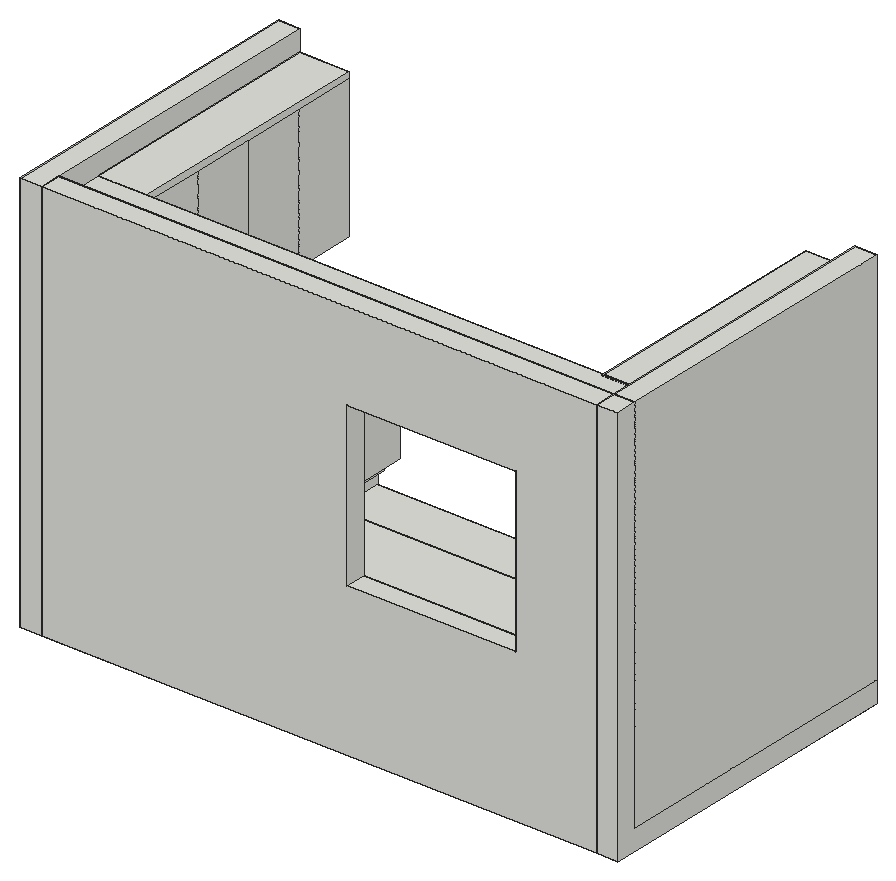
# SketchUp Ruby script. Lengths in inches.
U = 1.inch
M = Sketchup.active_model
def pt(a) = Geom::Point3d.new(a.map { |v| v * U })
def face(e, loops, mat)
  f = e.add_face(loops[0].map { |a| pt(a) })
  loops[1..].each { |l| e.add_face(l.map { |a| pt(a) }).erase! }
  f.material = f.back_material = mat if mat
  f
end
# faces: each face lists its corners as indices into pts; further lists are holes
def faces(e, pts, list, mat = nil) = list.each { |f| face(e, (f[0].is_a?(Array) ? f : [f]).map { |l| l.map { |i| pts[i] } }, mat) }
# xy, xz, yz: faces in a plane at the given z, y or x. An outline is a flat list of corners, or four numbers for a rectangle; further outlines are holes
def ring(l) = l.size == 4 ? [[l[0], l[1]], [l[2], l[1]], [l[2], l[3]], [l[0], l[3]]] : l.each_slice(2).to_a
def flat(e, list, mat, &to3) = list.each { |f| face(e, (f[0].is_a?(Array) ? f : [f]).map { |l| ring(l).map { |u, v| to3.(u, v) } }, mat) }
def xy(e, z, list, mat = nil) = flat(e, list, mat) { |x, y| [x, y, z] }
def xz(e, y, list, mat = nil) = flat(e, list, mat) { |x, z| [x, y, z] }
def yz(e, x, list, mat = nil) = flat(e, list, mat) { |y, z| [x, y, z] }
def lines(e, pts, list) = list.each { |a, b| e.add_line(pt(pts[a]), pt(pts[b])) }
# prism: a flat outline (further loops are holes) pulled along v
def prism(e, loops, v, mat = nil)
  f = face(e, loops, mat); d = Geom::Vector3d.new(v.map { |x| x * U })
  f.pushpull(f.normal.samedirection?(d) ? d.length : -d.length)
end
def box(e, o, s, mat = nil) = prism(e, [[o, [o[0] + s[0], o[1], o[2]], [o[0] + s[0], o[1] + s[1], o[2]], [o[0], o[1] + s[1], o[2]]]], [0, 0, s[2]], mat)
def at(x, y, z, deg = 0) = Geom::Transformation.translation(pt([x, y, z])) * Geom::Transformation.rotation(ORIGIN, Z_AXIS, deg.degrees)
def axes(o, x, y, z) = Geom::Transformation.new([*x, 0, *y, 0, *z, 0, *pt(o).to_a, 1])
def part(name) = M.definitions.add(name)
# library, detail: a bought-in or finely detailed component or shape, given as its bounding box
def library(name, o, s) = part(name).tap { |d| box(d.entities, o, s) }
def detail(e, o, s) = box(e.add_group.entities, o, s)
def put(e, d, t, mat = nil) = e.add_instance(d, t).tap { |i| i.material = mat if mat }
def group(e, t, mat = nil) = e.add_group.tap { |g| g.transformation = t; g.material = mat if mat }.entities
root = M.entities
c1 = part("A$C2FDA71ED")
p = [[230.9,-4.84,0],[210.9,-4.84,0],[210.9,15.16,0],[230.9,15.16,0],[118.17,5.52,0],[156.81,-4.84,0],
  [161.99,14.48,0],[123.35,24.84,0],[-230.9,-4.84,0],[-210.9,-4.84,0],[-210.9,15.16,0],[-230.9,15.16,0],
  [-118.17,5.52,0],[-156.81,-4.84,0],[-161.99,14.48,0],[-123.35,24.84,0],[323.64,5.52,0],[285,-4.84,0],
  [279.82,14.48,0],[318.46,24.84,0],[-323.64,5.52,0],[-285,-4.84,0],[-279.82,14.48,0],[-318.46,24.84,0],
  [-375,-24.84,0],[375,-24.84,0],[375,-4.84,0],[-375,-4.84,0]]
lines(c1.entities,p,[[0,1],[1,2],[2,3],[3,0],[4,5],[5,6],[6,7],[7,4],[8,9],[9,10],[10,11],[11,8],
  [12,13],[13,14],[14,15],[15,12],[16,17],[17,18],[18,19],[19,16],[20,21],[21,22],[22,23],[23,20],
  [24,25],[25,26],[26,27],[27,24]])
xy(root,0,[[6,29.29,28.03,30],[141.47,29.29,163.5,30]])
xy(root,4,[[32,20.3125,32,29.29,32.12,29.29,32.12,30,51.38,30,51.38,20.3125],[51.38,20.3125,51.5,29.29],[51.5,20.3125,59.75,30],[59.75,20.3125,91.5,30],[91.5,20.3125,92,30],
  [102,20.3125,116,30],[28.03,29.29,30,30],[30,29.29,32,30],[137.5,29.29,139.5,30]])
xy(root,17.27,[[51.77,29.29,91.23,30]])
xy(root,17.73,[[51.77,29.29,91.23,30]])
xy(root,25,[[51.5,29.29,91.5,30]])
xy(root,25.12,[[51.5,29.29,91.5,30]])
xy(root,32,[[30,29.29,32,30],[32.12,29.29,51.38,30],[51.5,29.29,91.5,30],[91.5,29.29,102,30],[102,29.29,139.5,30]])
xy(root,32.8,[[6,6,32,29.29],[32,6,163.5,29.29],[6,29.29,29.29,30],[29.29,29.29,139.5,30],[139.5,29.29,163.5,30]])
xy(root,34,[[6,6,163.5,30]])
xy(root,100,[[6,19.29,20,20],[35.75,19.29,51.5,20],[51.5,19.29,71.5,20],[71.5,19.29,91.5,20],[149.5,19.29,163.5,20],
  [149.5,20,150.21,21.97]])
xy(root,100.12,[[6,6,163.5,19.29],[6,19.29,163.5,20],[149.5,20,150.21,91.5]])
xy(root,102,[[6,6,163.5,20]])
xz(root,6,[[6,32.8,163.5,34],[6,100.12,163.5,102]])
xz(root,19.29,[[6,100,163.5,100.12]])
xz(root,20,[[150.21,100,163.5,100.12],[6,100.12,163.5,102]])
xz(root,20.3125,[[32,0,137.5,4]])
xz(root,29.29,[[6,0,28.03,0,28.03,4,30,4,30,32,29.29,32,29.29,32.8,6,32.8],[28.03,0,30,4],[141.47,0,141.47,4,139.5,4,139.5,32,29.29,32,29.29,32.8,163.5,32.8,151.5,16.4,163.5,0],[139.5,0,141.47,4],[32,4,32.12,32],
  [51.38,4,51.5,32],[51.77,17.27,91.23,17.73],[51.5,25,91.5,25.12]])
xz(root,30,[[6,0,6,32.8,29.29,32.8,29.29,32,30,32,30,4,28.03,4,28.03,0],[30,4,32,32],[32.12,4,51.38,32],[51.5,4,91.5,17],[137.5,4,139.5,32],
  [[51.5,17,91.5,18],[51.77,17.27,91.23,17.73]],[51.5,18,91.5,25],[51.5,25.12,91.5,32],[6,32.8,163.5,34]])
yz(root,6,[[29.29,0,30,32.8],[6,32.8,30,34],[19.29,100,20,100.12],[6,100.12,20,102]])
yz(root,28.03,[[29.29,0,30,4]])
yz(root,30,[[29.29,4,30,32]])
yz(root,32,[[29.29,4,30,32]])
yz(root,32.12,[[29.29,4,30,32]])
yz(root,51.38,[[29.29,4,30,32]])
yz(root,51.5,[[29.29,4,30,17],[29.29,17,30,18],[29.29,18,30,25],[29.29,25.12,30,32]])
yz(root,51.77,[[29.29,17.27,30,17.73]])
yz(root,91.23,[[29.29,17.27,30,17.73]])
yz(root,91.5,[[29.29,25,30,25.12]])
yz(root,139.5,[[29.29,4,30,32]])
yz(root,150.21,[[20,100,91.5,100.12]])
yz(root,163.5,[[6,32.8,30,34],[19.29,100,20,100.12],[6,100.12,20,102]])
p = [[151.5,30,16.4],[163.5,30,0],[163.5,29.29,0],[151.5,29.29,16.4],[163.5,30,32.8],[163.5,29.29,32.8],
  [6115.93,1751.17,0],[6115.93,1779.17,0],[6091.93,1751.17,0],[6091.93,1779.17,0],[6738.71,1689.96,0],[6800.21,1689.96,0],
  [6738.71,1693.96,0],[6756.71,1693.96,0],[6738.71,1723.96,0],[6774.71,1723.96,0],[6738.71,1722.76,0],[6774.71,1722.76,0],
  [6738.71,1721.96,0],[6756.71,1721.96,0],[6800.21,1723.96,0],[6800.21,1693.96,0],[6824.21,1723.96,0],[6824.21,1689.96,0],
  [6798.21,1723.96,0],[6798.21,1722.76,0],[6812.21,1706.96,0],[6738.71,1749.96,0],[6738.71,1791.96,0],[6756.58,1791.96,0],
  [6824.21,1791.96,0],[6824.21,1749.96,0],[6810.21,1791.96,0],[6810.21,1749.96,0],[6817.21,1770.96,0],[6738.71,1803.96,0],
  [6824.21,1803.96,0],[6756.58,1749.96,0],[6774.46,1749.96,0],[6774.46,1791.96,0],[6792.33,1749.96,0],[6792.33,1791.96,0],
  [6774.71,1693.96,0],[6774.71,1721.96,0],[6798.21,1721.96,0],[6798.21,1693.96,0],[29.29,30,32],[29.29,29.29,32],
  [20,37.99,100],[20,37.99,60],[20,37.875,100],[20,55.87,60],[20,55.87,100],[20,37.875,60],
  [20,91.5,100],[20,55.75,100],[20,55.75,60],[141.5,6,36],[141.5,6,84],[140.5,6,37],
  [140.5,6,83],[92.5,6,37],[92.5,6,83],[102,30,4],[102,30,17],[137.5,30,18],
  [102,30,18],[137.5,30,17],[137.5,6,84],[91.5,6,84],[91.5,6,36],[102,30,32],
  [92,30,4],[30,91.5,34],[29.29,91.5,34],[30,30,34],[32,29.29,0],[32,20.3125,0],
  [137.5,29.29,0],[137.5,20.3125,0],[137.5,29.29,4],[137.5,20.3125,4],[149.5,22.09,100],[149.5,22.09,58],
  [149.5,21.97,58],[149.5,21.97,100],[149.5,91.5,100],[150.21,91.5,100],[150.21,22.09,100],[30,29.29,0],
  [139.5,29.29,0]]
faces(root,p,[[0,1,2,3],[4,0,3,5]])
lines(root,p,[[6,7],[8,9],[10,11],[12,13],[10,12],[14,15],[16,17],[18,19],[20,21],[22,23],[24,25],[15,17],
  [22,26],[20,26],[14,27],[28,29],[30,31],[32,33],[30,34],[32,34],[28,35],[35,36],[36,30],[37,29],
  [38,39],[40,41],[19,13],[11,23],[13,42],[16,14],[18,16],[12,18],[15,24],[17,25],[43,44],[19,43],
  [21,11],[25,44],[43,42],[17,43],[26,11],[26,23],[27,28],[37,38],[29,39],[31,22],[34,33],[34,31],
  [37,27],[42,45],[24,20],[44,45],[38,40],[39,41],[45,21],[20,22],[40,33],[41,32],[33,31],[32,30],
  [46,47],[48,49],[48,50],[51,52],[50,53],[54,52],[55,48],[55,56],[57,58],[59,60],[61,59],[60,62],
  [63,64],[65,66],[67,64],[68,69],[70,57],[62,61],[58,68],[64,66],[69,70],[66,71],[63,72],[4,1],
  [73,74],[75,73],[76,77],[78,79],[80,81],[82,83],[83,84],[84,85],[86,82],[86,87],[82,88],[76,89],
  [90,78]])
put(root,c1,axes([6341.85,1603.75,0],[0.83336,0,0],[0,0.83336,0],[0,0,0.83336]))
g1 = group(root,at(163.5,91.5,60))
xy(g1,-2,[[-14,-72.21,-14,-69.53,-13.29,-69.53,-13.29,-69.41,-14,-69.41,-14,-53.74,-13.29,-53.74,-13.29,-53.625,-14,-53.625,-14,-35.75,-13.29,-35.75,-13.29,-35.63,-14,-35.63,-14,-17.875,-13.29,-17.875,-13.29,0,0,0,0,-72.21],[-14,-17.76,-13.29,0]])
xy(g1,40,[[-14,-71.5,-13.29,-69.53],[-14,-69.41,-13.29,-53.74],[-14,-53.625,-13.29,-35.75],[-14,-35.63,-13.29,-17.875],[-14,-17.76,-13.29,0]])
xy(g1,40.12,[[-14,-71.5,-13.29,0]])
xy(g1,42,[[-14,-72.21,0,0]])
xz(g1,-72.21,[[-14,-2,0,42]])
xz(g1,-71.5,[[-14,40,-13.29,40.12]])
xz(g1,-69.53,[[-14,-2,-13.29,40]])
xz(g1,-69.41,[[-14,-2,-13.29,40]])
xz(g1,-53.74,[[-14,-2,-13.29,40]])
xz(g1,-53.625,[[-14,-2,-13.29,40]])
xz(g1,-35.75,[[-14,-2,-13.29,40]])
xz(g1,-35.63,[[-14,-2,-13.29,40]])
xz(g1,-17.875,[[-14,-2,-13.29,40]])
xz(g1,-17.76,[[-14,-2,-13.29,40]])
xz(g1,0,[[-13.29,-2,-13.29,40.12,-14,40.12,-14,42,0,42,0,-2],[-14,-2,-13.29,40]])
yz(g1,-14,[[-72.21,-2,-69.53,40],[-69.41,-2,-53.74,40],[-53.625,-2,-35.75,40],[-35.63,-2,-17.875,40],[-17.76,-2,0,40],
  [-72.21,40,-72.21,42,0,42,0,40.12,-71.5,40.12,-71.5,40]])
yz(g1,-13.29,[[-69.53,-2,-69.41,40],[-53.74,-2,-53.625,40],[-35.75,-2,-35.63,40],[-17.875,-2,-17.76,40],[-17.76,-2,0,40],
  [-71.5,40,0,40.12]])
yz(g1,0,[[-72.21,-2,0,42]])
g2 = group(root,at(139.5,6,0))
xy(g2,0,[[-109.5,0,0,23.29]])
xy(g2,4,[[-109.5,23.29,-107.5,24],[-47.88,23.29,-37.62,24],[-37.5,23.29,-2.12,24],[-2,23.29,0,24]])
xy(g2,17.27,[[-37.23,23.29,-2.38,24]])
xy(g2,17.73,[[-37.23,23.29,-2.38,24]])
xy(g2,25.12,[[-88,23.29,-48,24]])
xy(g2,32,[[-109.5,23.29,-107.5,24],[-88,23.29,-48,24],[-47.88,23.29,-37.62,24],[-37.5,23.29,-2.12,24],[-2,23.29,0,24]])
xy(g2,32.8,[[-109.5,0,0,23.29]])
xz(g2,0,[[-109.5,0,0,32.8]])
xz(g2,23.29,[[-109.5,0,0,4],[-107.5,4,-88,32],[-88,4,-48,25],[-48,4,-47.88,32],[-37.62,4,-37.5,32],
  [-2.12,4,-2,32],[-37.23,17.27,-2.38,17.73],[-88,25,-48,25.12]])
xz(g2,24,[[-109.5,4,-107.5,32],[-47.88,4,-37.62,32],[-37.5,4,-2.12,17],[-2,4,0,32],[[-37.5,17,-2.12,18],[-37.23,17.27,-2.38,17.73]],
  [-37.5,18,-2.12,32],[-88,25.12,-48,32]])
yz(g2,-107.5,[[23.29,4,24,32]])
yz(g2,-88,[[23.29,25.12,24,32]])
yz(g2,-48,[[23.29,25.12,24,32]])
yz(g2,-47.88,[[23.29,4,24,32]])
yz(g2,-37.62,[[23.29,4,24,32]])
yz(g2,-37.5,[[23.29,4,24,32]])
yz(g2,-37.23,[[23.29,17.27,24,17.73]])
yz(g2,-2.38,[[23.29,17.27,24,17.73]])
yz(g2,-2.12,[[23.29,4,24,32]])
yz(g2,-2,[[23.29,4,24,32]])
yz(g2,0,[[0,0,0,32.8,23.29,32.8,23.29,32,24,32,24,4,23.29,4,23.29,0]])
g3 = group(root,at(91.5,20,60))
xy(g3,-2,[[50,-14,58,-14,58,0,56.03,0,56.03,-0.71,55.91,-0.71,55.91,0,50,0]])
xy(g3,0,[[-71.5,-14,0,-14,0,0,-19.88,0,-19.88,-0.71,-20,-0.71,-20,0,-40,0,-40,-0.71,-40.12,-0.71,-40.12,0,-55.63,0,-55.63,-0.71,-55.75,-0.71,-55.75,0,-69.41,0,-69.41,-0.71,-69.53,-0.71,-69.53,0,-71.5,0]])
xy(g3,24,[[0,-14,50,-14,50,-0.71,49.88,-0.71,49.88,0,0.12,0,0.12,-0.71,0,-0.71]])
xy(g3,40,[[-71.5,-14,-71.5,0,-69.53,0,-69.53,-0.71,-69.41,-0.71,-69.41,0,-55.75,0,-55.75,-0.71,-55.63,-0.71,-55.63,0,-40.12,0,-40.12,-0.71,-40,-0.71,-40,0,-20,0,-20,-0.71,-19.88,-0.71,-19.88,0,0,0,0,-0.71,0.12,-0.71,0.12,0,49.88,0,49.88,-0.71,50,-0.71,50,0,55.91,0,55.91,-0.71,56.03,-0.71,56.03,0,58,0,58,-14]])
xz(g3,-14,[[50,-2,50,24,0,24,0,0,-71.5,0,-71.5,40,58,40,58,-2]])
xz(g3,-0.71,[[55.91,-2,56.03,40],[-69.53,0,-69.41,40],[-55.75,0,-55.63,40],[-40.12,0,-40,40],[-20,0,-19.88,40],
  [0,24,0.12,40],[49.88,24,50,40]])
xz(g3,0,[[50,-2,55.91,40],[56.03,-2,58,40],[-71.5,0,-69.53,40],[-69.41,0,-55.75,40],[-55.63,0,-40.12,40],
  [-40,0,-20,40],[-19.88,0,0,40],[0.12,24,49.88,40]])
yz(g3,-71.5,[[-14,0,0,40]])
yz(g3,-69.53,[[-0.71,0,0,40]])
yz(g3,-69.41,[[-0.71,0,0,40]])
yz(g3,-55.75,[[-0.71,0,0,40]])
yz(g3,-55.63,[[-0.71,0,0,40]])
yz(g3,-40.12,[[-0.71,0,0,40]])
yz(g3,-40,[[-0.71,0,0,40]])
yz(g3,-20,[[-0.71,0,0,40]])
yz(g3,-19.88,[[-0.71,0,0,40]])
yz(g3,0,[[-14,0,0,24],[-0.71,24,0,40]])
yz(g3,0.12,[[-0.71,24,0,40]])
yz(g3,49.88,[[-0.71,24,0,40]])
yz(g3,50,[[-14,-2,0,24],[-0.71,24,0,40]])
yz(g3,55.91,[[-0.71,-2,0,40]])
yz(g3,56.03,[[-0.71,-2,0,40]])
yz(g3,58,[[-14,-2,0,40]])
g4 = group(root,at(163.5,6,58))
box(g4,[-14,0,0],[14,14,42])
box(g4,[-157.5,0,2],[14,14,40])
g5 = group(root,at(6,91.5,60,-90))
xy(g5,0,[[0,0,0,13.29,17.82,13.29,17.82,14,35.63,14,35.63,13.29,35.75,13.29,35.75,14,53.51,14,53.51,13.29,53.625,13.29,53.625,14,69.41,14,69.41,13.29,69.53,13.29,69.53,14,71.5,14,71.5,0],[0,13.29,17.7,14]])
xy(g5,40,[[0,13.29,17.7,14],[17.82,13.29,35.63,14],[35.75,13.29,53.51,14],[53.625,13.29,69.41,14],[69.53,13.29,71.5,14]])
xy(g5,40.12,[[0,13.29,71.5,14]])
xy(g5,42,[[0,0,71.5,14]])
xz(g5,0,[[0,0,71.5,42]])
xz(g5,13.29,[[0,0,17.7,40],[17.7,0,17.82,40],[53.51,0,53.625,40],[69.41,0,69.53,40],[0,40,71.5,40.12]])
xz(g5,14,[[0,0,17.7,40],[17.82,0,35.63,40],[35.75,0,53.51,40],[53.625,0,69.41,40],[69.53,0,71.5,40],
  [0,40.12,71.5,42]])
yz(g5,0,[[0,0,0,42,14,42,14,40.12,13.29,40.12,13.29,0],[13.29,0,14,40]])
yz(g5,17.7,[[13.29,0,14,40]])
yz(g5,17.82,[[13.29,0,14,40]])
yz(g5,35.63,[[13.29,0,14,40]])
yz(g5,35.75,[[13.29,0,14,40]])
yz(g5,53.51,[[13.29,0,14,40]])
yz(g5,53.625,[[13.29,0,14,40]])
yz(g5,69.41,[[13.29,0,14,40]])
yz(g5,69.53,[[13.29,0,14,40]])
yz(g5,71.5,[[0,0,14,0,14,40,13.29,40,13.29,40.12,14,40.12,14,42,0,42]])
g6 = group(root,at(6,6,-6))
prism(g6,[[[0,0,114],[0,0,0],[157.5,0,0],[157.5,0,114]],[[134.5,0,89],[134.5,0,43],[86.5,0,43],[86.5,0,89]]],[0,-6,0])
g7 = group(root,at(6,30,0))
xy(g7,0,[[0,0,22.03,61.5]])
xy(g7,4,[[22.03,0,24,2],[22.03,2,23.29,31.75],[23.29,2.12,24,31.75],[22.03,31.75,23.29,61.5],[23.29,31.87,24,61.5]])
xy(g7,17,[[23.29,2.12,24,31.75],[23.29,31.75,24,31.87],[23.29,31.87,24,61.5]])
xy(g7,17.27,[[23.29,2.38,24,31.75],[23.29,31.75,24,61.23]])
xy(g7,17.73,[[23.29,2.38,24,31.75],[23.29,31.75,24,61.23]])
xy(g7,18,[[23.29,2.12,24,31.75],[23.29,31.75,24,31.87],[23.29,31.87,24,61.5]])
xy(g7,32,[[23.29,0,24,2],[23.29,2.12,24,31.75],[23.29,31.87,24,61.5]])
xy(g7,32.8,[[23.29,0,24,2],[23.29,2,24,61.5]])
xy(g7,34,[[0,0,24,61.5]])
xz(g7,0,[[0,0,22.03,0,22.03,4,24,4,24,32,23.29,32,23.29,32.8,24,32.8,24,34,0,34]])
xz(g7,2,[[23.29,4,24,17],[23.29,17,24,18],[23.29,18,24,32]])
xz(g7,2.12,[[23.29,4,24,17],[23.29,17,24,18],[23.29,18,24,32]])
xz(g7,2.38,[[23.29,17.27,24,17.73]])
xz(g7,31.75,[[23.29,4,24,17],[23.29,18,24,32]])
xz(g7,31.87,[[23.29,4,24,17],[23.29,18,24,32]])
xz(g7,61.23,[[23.29,17.27,24,17.73]])
xz(g7,61.5,[[0,0,0,34,24,34,24,32.8,23.29,32.8,23.29,18,24,18,24,17,23.29,17,23.29,4,22.03,4,22.03,0],[23.29,4,24,17],[23.29,18,24,32]])
yz(g7,0,[[0,0,61.5,34]])
yz(g7,22.03,[[0,0,61.5,4]])
yz(g7,23.29,[[2,4,2.12,17],[2.12,4,31.75,17],[31.75,4,31.87,17],[31.87,4,61.5,17],[2,17,2.12,18],
  [2.38,17.27,61.23,17.73],[2,18,2.12,32],[2.12,18,31.75,32],[31.75,18,31.87,32],[31.87,18,61.5,32],
  [0,32,61.5,32.8]])
yz(g7,24,[[0,4,2,32],[2.12,4,31.75,17],[31.87,4,61.5,17],[[2.12,17,61.5,18],[2.38,17.27,61.23,17.73]],[2.12,18,31.75,32],
  [31.87,18,61.5,32],[0,32.8,61.5,34]])
g8 = group(root,at(163.5,91.5,0))
xy(g8,0,[[-22.03,-61.5,-18,0]])
xy(g8,4,[[-24,-61.5,-22.03,-61.5,-22.03,0,-24,0,-24,-17.88,-23.29,-17.88,-23.29,-18,-24,-18,-24,-36,-23.29,-36,-23.29,-36.12,-24,-36.12,-24,-59.38,-23.29,-59.38,-23.29,-59.5,-24,-59.5]])
xy(g8,32,[[-24,-61.5,-23.29,-59.5],[-24,-59.38,-23.29,-36.12],[-24,-36,-23.29,-18],[-24,-17.88,-23.29,0]])
xy(g8,32.8,[[-24,-61.5,-23.29,0]])
xy(g8,34,[[-24,-61.5,-23.29,0]])
xz(g8,-61.5,[[-22.03,0,-22.03,4,-24,4,-24,32,-23.29,32,-23.29,34,-18,34,-18,0],[-24,32.8,-23.29,34]])
xz(g8,-59.5,[[-24,4,-23.29,32]])
xz(g8,-59.38,[[-24,4,-23.29,32]])
xz(g8,-36.12,[[-24,4,-23.29,32]])
xz(g8,-36,[[-24,4,-23.29,32]])
xz(g8,-18,[[-24,4,-23.29,32]])
xz(g8,-17.88,[[-24,4,-23.29,32]])
xz(g8,0,[[-24,4,-23.29,32],[-24,32.8,-23.29,34]])
yz(g8,-24,[[-61.5,4,-59.5,32],[-59.38,4,-36.12,32],[-36,4,-18,32],[-17.88,4,0,32],[-61.5,32.8,0,34]])
yz(g8,-23.29,[[-61.5,32,0,32.8],[-61.5,32.8,0,34]])
yz(g8,-22.03,[[-61.5,0,0,4]])
g9 = group(g8,at(-24,0,0))
xy(g9,0,[[1.97,-61.5,24,0]])
xy(g9,4,[[0.71,-61.5,1.97,0]])
xy(g9,34,[[0.71,-61.5,24,0]])
xz(g9,-61.5,[[1.97,0,1.97,4,0.71,4,0.71,34,24,34,24,0]])
xz(g9,0,[[1.97,0,24,0,24,34,0.71,34,0.71,4,1.97,4]])
yz(g9,0.71,[[-61.5,4,-36.12,4,-36.12,32,-36,32,-36,4,-18,4,-18,32,-17.88,32,-17.88,4,0,4,0,34,-61.5,34],[-36.12,4,-36,32],[-18,4,-17.88,32]])
yz(g9,1.97,[[-61.5,0,0,4]])
yz(g9,24,[[-61.5,0,0,34]])
p = [[0.71,0,34],[0,0,34]]
lines(g9,p,[[0,1]])
g10 = group(root,at(6,30,-6))
xy(g10,0,[[-6,-30,0,61.5],[157.5,-30,163.5,61.5],[0,-24,157.5,61.5]])
xy(g10,6,[[0,-24,157.5,61.5],[157.5,-24,163.5,61.5]])
xy(g10,114,[[-6,-30,0,61.5],[157.5,-30,163.5,-24],[157.5,-24,163.5,61.5]])
xz(g10,-30,[[-6,0,0,114],[157.5,0,163.5,114]])
xz(g10,-24,[[0,0,157.5,6],[157.5,6,163.5,114]])
xz(g10,61.5,[[-6,0,0,6],[0,0,157.5,6],[157.5,0,163.5,6],[-6,6,0,114],[157.5,6,163.5,114]])
yz(g10,-6,[[-30,0,61.5,6],[-30,6,61.5,114]])
yz(g10,0,[[-30,0,-24,6],[-24,0,61.5,6],[-30,6,61.5,114]])
yz(g10,157.5,[[-30,0,-24,114],[-24,0,61.5,6],[-24,6,61.5,114]])
yz(g10,163.5,[[-30,0,-30,114,-24,114,-24,6,61.5,6,61.5,0],[-24,6,61.5,114]])
